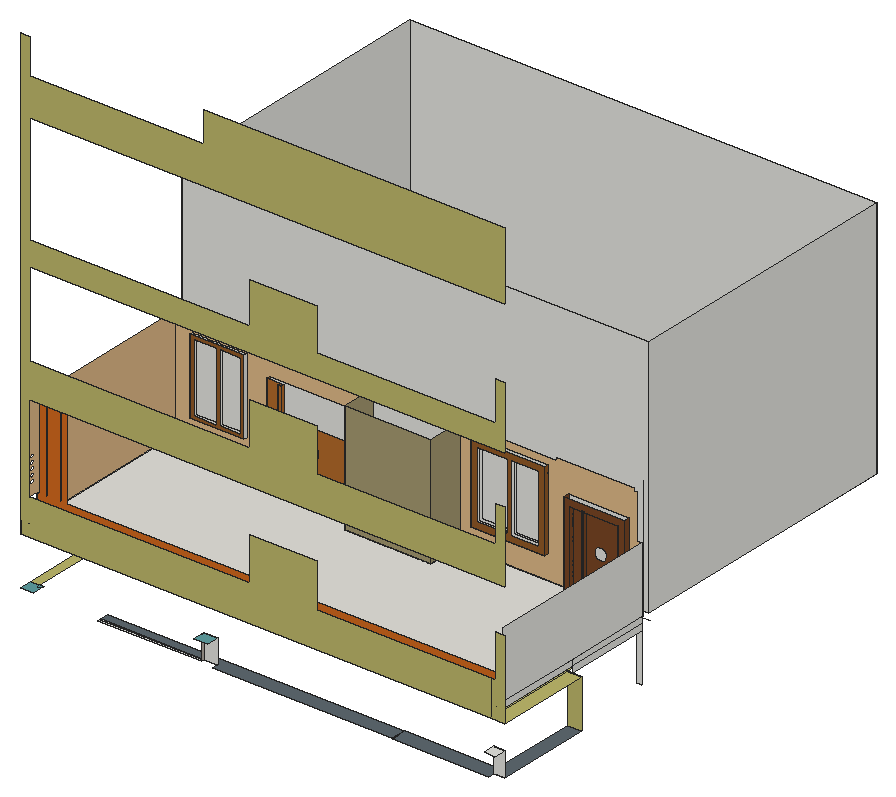
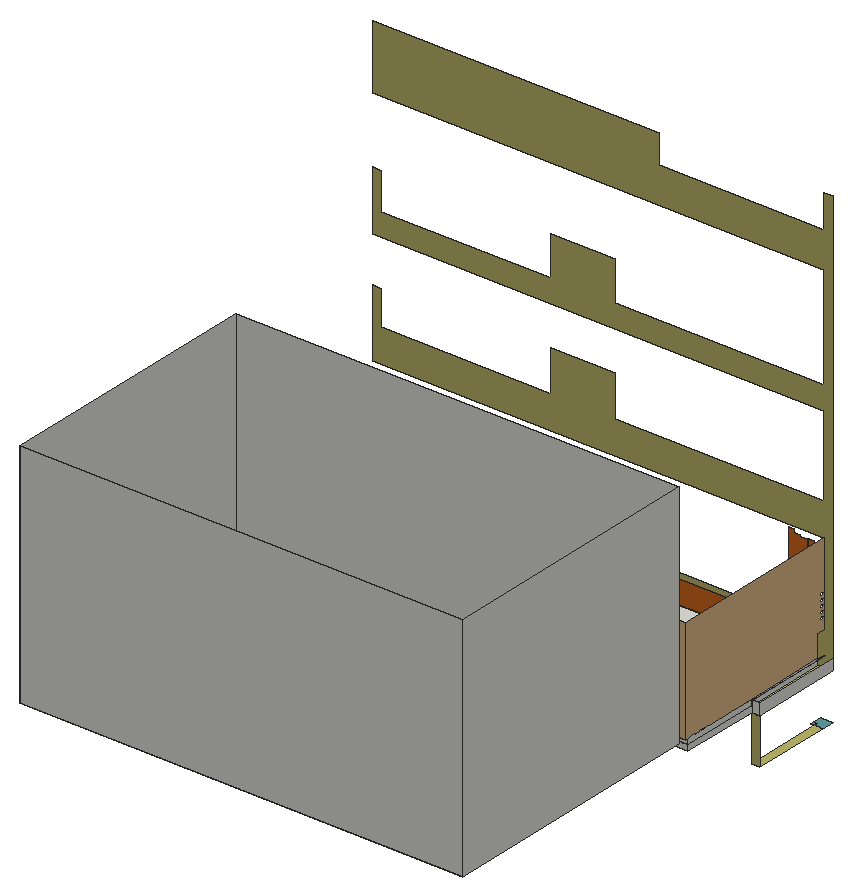
# SketchUp Ruby script. Lengths in inches.
U = 1.inch
M = Sketchup.active_model
def pt(a) = Geom::Point3d.new(a.map { |v| v * U })
def face(e, loops, mat)
  f = e.add_face(loops[0].map { |a| pt(a) })
  loops[1..].each { |l| e.add_face(l.map { |a| pt(a) }).erase! }
  f.material = f.back_material = mat if mat
  f
end
# faces: each face lists its corners as indices into pts; further lists are holes
def faces(e, pts, list, mat = nil) = list.each { |f| face(e, (f[0].is_a?(Array) ? f : [f]).map { |l| l.map { |i| pts[i] } }, mat) }
# xy, xz, yz: faces in a plane at the given z, y or x. An outline is a flat list of corners, or four numbers for a rectangle; further outlines are holes
def ring(l) = l.size == 4 ? [[l[0], l[1]], [l[2], l[1]], [l[2], l[3]], [l[0], l[3]]] : l.each_slice(2).to_a
def flat(e, list, mat, &to3) = list.each { |f| face(e, (f[0].is_a?(Array) ? f : [f]).map { |l| ring(l).map { |u, v| to3.(u, v) } }, mat) }
def xy(e, z, list, mat = nil) = flat(e, list, mat) { |x, y| [x, y, z] }
def xz(e, y, list, mat = nil) = flat(e, list, mat) { |x, z| [x, y, z] }
def yz(e, x, list, mat = nil) = flat(e, list, mat) { |y, z| [x, y, z] }
def lines(e, pts, list) = list.each { |a, b| e.add_line(pt(pts[a]), pt(pts[b])) }
# prism: a flat outline (further loops are holes) pulled along v
def prism(e, loops, v, mat = nil)
  f = face(e, loops, mat); d = Geom::Vector3d.new(v.map { |x| x * U })
  f.pushpull(f.normal.samedirection?(d) ? d.length : -d.length)
end
def box(e, o, s, mat = nil) = prism(e, [[o, [o[0] + s[0], o[1], o[2]], [o[0] + s[0], o[1] + s[1], o[2]], [o[0], o[1] + s[1], o[2]]]], [0, 0, s[2]], mat)
def at(x, y, z, deg = 0) = Geom::Transformation.translation(pt([x, y, z])) * Geom::Transformation.rotation(ORIGIN, Z_AXIS, deg.degrees)
def axes(o, x, y, z) = Geom::Transformation.new([*x, 0, *y, 0, *z, 0, *pt(o).to_a, 1])
def part(name) = M.definitions.add(name)
# library, detail: a bought-in or finely detailed component or shape, given as its bounding box
def library(name, o, s) = part(name).tap { |d| box(d.entities, o, s) }
def detail(e, o, s) = box(e.add_group.entities, o, s)
def put(e, d, t, mat = nil) = e.add_instance(d, t).tap { |i| i.material = mat if mat }
def group(e, t, mat = nil) = e.add_group.tap { |g| g.transformation = t; g.material = mat if mat }.entities
root = M.entities
M.materials.add("[0036_BurlyWood]").color = [222, 184, 135]
M.materials.add("[0041_Chocolate]").color = [210, 105, 30]
M.materials.add("[0057_DarkKhaki]").color = [189, 183, 107]
M.materials.add("[0081_CadetBlue]").color = [95, 158, 160]
M.materials.add("[Formica Speckled Grey]").color = [94, 105, 111]
M.materials.add("[Marble Carrara Gold Floor Tile]").color = [225, 223, 217]
M.materials.add("[Stone Masonry Multi]").color = [182, 175, 164]
M.materials.add("[Translucent Glass Blue]").color = [100, 149, 237]
M.materials["[Translucent Glass Blue]"].alpha = 0.5
M.materials.add("[Wood Bamboo]").color = [177, 105, 43]
M.materials.add("[Wood Floor Parquet]").color = [145, 89, 39]
M.materials.add("[Wood Lumber ButtJoined]").color = [164, 152, 112]
M.materials.add("[Wood Veneer 01]").color = [120, 70, 37]
xy(root,60,[[373.99,6,374.05,12],[79.49,9,181.875,11.375],[79.49,11.375,181.875,12]])
xy(root,60,[[0,24.5,9,106.65]],"[0057_DarkKhaki]")
xy(root,60,[[0,12,12.93,12,12.93,21,9,21,9,24.5,0,24.5],[9,21,12.93,24.5]],"[0081_CadetBlue]")
xy(root,60,[[195.69,6,372.4375,6,372.4375,21,79.49,21,79.49,12,195.69,12],[374.05,6,469.21,6,469.21,12,480,12,480,106.65,466.21,106.65,466.21,21,373.99,21,373.99,12,374.05,12]],"[Formica Speckled Grey]")
xy(root,75.62,[[308.99,189.3,366.74,192.3]])
xy(root,78.62,[[337.87,189.3,341.25,192.3]])
xy(root,78.62,[[311.99,189.3,337.87,192.3],[341.25,189.3,363.74,192.3]],"[Wood Floor Parquet]")
xy(root,84,[[469.21,0,480,12],[246.91,192.3,282.91,196.8]])
xy(root,84,[[181.875,0,195.69,12]],"[0081_CadetBlue]")
xy(root,84,[[246.91,189.3,282.91,192.3]],"[Wood Veneer 01]")
xy(root,88.67,[[242.24,189.3,287.58,192.3]],"[Wood Veneer 01]")
xy(root,89.97,[[341.25,189.3,363.74,192.3]])
xy(root,89.97,[[311.99,189.3,337.87,192.3]],"[Wood Floor Parquet]")
xy(root,92.64,[[311.99,189.3,337.87,192.3],[341.25,189.3,363.74,192.3]],"[Wood Floor Parquet]")
xy(root,101.31,[[337.87,189.3,341.25,192.3],[341.25,189.3,363.74,192.3]])
xy(root,101.31,[[311.99,189.3,337.87,192.3]],"[Wood Floor Parquet]")
xy(root,104.31,[[308.99,189.3,366.74,192.3]])
xy(root,105.6875,[[413.91,189.3,439.47,192.3]],"[Wood Floor Parquet]")
xy(root,108,[[205.37,156.87,290.8125,192.3]])
xy(root,108,[[0,12,0,106.65,9,106.65,9,189.3,90.1,189.3,90.1,186.3,99.83,186.3,99.83,189.3,103.48,189.3,103.48,186.3,113.21,186.3,113.21,189.3,115.97,189.3,115.97,186.3,128.46,186.3,128.46,189.3,186.5,189.3,186.5,192.3,205.37,192.3,205.37,156.87,290.8125,156.87,290.8125,192.3,398.79,192.3,398.79,186.3,405.17,186.3,405.17,189.3,416.3125,189.3,416.3125,186.3,418.65,186.3,418.65,189.3,452.54,189.3,452.54,186.3,458.79,186.3,458.79,192.3,466.21,192.3,466.21,12],[466.21,12,480,106.65]],"[0057_DarkKhaki]")
xy(root,108.6875,[[410.91,189.3,442.47,192.3]])
xy(root,114.1875,[[9,21,471,21,471,192.3,458.79,192.3,458.79,186.3,452.54,186.3,452.54,189.3,418.65,189.3,418.65,186.3,416.3125,186.3,416.3125,189.3,405.17,189.3,405.17,186.3,398.79,186.3,398.79,192.3,290.8125,192.3,290.8125,156.87,205.37,156.87,205.37,192.3,186.5,192.3,186.5,189.3,128.46,189.3,128.46,186.3,115.97,186.3,115.97,189.3,113.21,189.3,113.21,186.3,103.48,186.3,103.48,189.3,99.83,189.3,99.83,186.3,90.1,186.3,90.1,189.3,9,189.3],[205.37,156.87,290.8125,192.3]])
xy(root,120,[[205.37,156.87,290.8125,192.3],[90.1,186.3,99.83,186.3,99.83,189.3,102.5,189.3,102.5,192.3,9,192.3,9,189.3,90.1,189.3],[103.48,186.3,113.21,189.3],[115.97,186.3,118.73,189.3],[118.73,186.3,119.35,189.3],
  [119.35,186.3,128.46,189.3],[398.79,186.3,405.17,192.3],[416.3125,186.3,418.65,186.3,418.65,189.3,452.54,189.3,452.54,192.3,405.17,192.3,405.17,189.3,416.3125,189.3],[452.54,186.3,458.79,192.3],[102.5,189.3,129,192.3],
  [129,189.3,186.5,192.3],[9,201.23,471,483]])
xy(root,120,[[9,21,471,21,471,192.3,458.79,192.3,458.79,186.3,452.54,186.3,452.54,189.3,418.65,189.3,418.65,186.3,416.3125,186.3,416.3125,189.3,405.17,189.3,405.17,186.3,398.79,186.3,398.79,192.3,290.8125,192.3,290.8125,156.87,205.37,156.87,205.37,192.3,186.5,192.3,186.5,189.3,128.46,189.3,128.46,186.3,115.97,186.3,115.97,189.3,113.21,189.3,113.21,186.3,103.48,186.3,103.48,189.3,99.83,189.3,99.83,186.3,90.1,186.3,90.1,189.3,9,189.3]],"[Marble Carrara Gold Floor Tile]")
xy(root,141.78,[[26.52,189.3,79.7,192.3]])
xy(root,143.29,[[303.94,192.3,377.89,195.3]])
xy(root,143.29,[[303.94,189.3,377.89,192.3]],"[Wood Floor Parquet]")
xz(root,12,[[181.875,60,195.69,84],[469.21,60,480,84]])
xz(root,12,[[0,108,466.21,108,466.21,144,293.97,144,293.97,186.625,227.54,186.625,227.54,144,9,144,9,229.6875,480,229.6875,480,300,471,300,471,264,293.97,264,293.97,306.625,227.54,306.625,227.54,264,9,264,9,348,480,348,480,410.4375,471.0625,410.4375,471.0625,372,293.97,372,293.97,413.38,227.54,413.38,227.54,372,9,372,9,480,480,480,480,547.59,181.625,547.59,181.625,517.1875,9,517.1875,9,552,0,552],[466.21,108,480,108,480,186.25,471,186.25,471,144,466.21,144]],"[0057_DarkKhaki]")
xz(root,21,[[9,114.1875,471,120]])
xz(root,21,[[9,120,9,144,12.36,144,12.36,229.6875,17.86,229.6875,17.86,144,20.11,144,20.11,229,25.61,229,25.61,144,26.86,144,26.86,229.6875,32.36,229.6875,32.36,144,33.61,144,33.61,233.5625,39.11,233.5625,39.11,144,471,144,471,120]],"[0041_Chocolate]")
xz(root,106.65,[[0,108,7.75,120],[7.75,108,9,120]])
xz(root,106.65,[[0,60,9,108],[466.21,60,480,108]],"[0057_DarkKhaki]")
xz(root,156.87,[[205.37,108,290.8125,114.1875],[205.37,114.1875,290.8125,120]])
xz(root,156.87,[[205.37,120,290.8125,229.6875]],"[Wood Lumber ButtJoined]")
xz(root,186.3,[[90.1,108,99.83,114.1875],[103.48,108,113.21,114.1875],[115.97,108,118.73,114.1875],[118.73,108,119.35,114.1875],[119.35,108,128.46,114.1875],
  [398.79,108,405.17,114.1875],[416.3125,108,418.65,114.1875],[452.54,108,458.79,114.1875],[90.1,114.1875,99.83,120],[103.48,114.1875,113.21,120],
  [115.97,114.1875,118.73,120],[118.73,114.1875,119.35,120],[119.35,114.1875,128.46,120],[398.79,114.1875,405.17,120],[416.3125,114.1875,418.65,120],
  [452.54,114.1875,458.79,120]])
xz(root,186.3,[[115.97,120,119.35,204],[144.0625,142.74,146.68,143.19,149.1,144.31,151.14,146.01,152.68,148.18,153.6,150.67,153.84,153.32,153.39,155.94,152.28,158.36,150.58,160.4,148.41,161.9375,145.91,162.86,143.26,163.1,140.64,162.65,138.23,161.54,136.18,159.84,134.65,157.67,133.73,155.17,133.48,152.52,133.93,149.9,135.05,147.49,136.75,145.44,138.92,143.91,141.41,142.99]],"[Wood Bamboo]")
xz(root,186.3,[[398.79,120,405.17,120,405.17,197.62,452.41,197.62,452.41,126.38,452.54,120,458.79,120,458.79,204,398.79,204],[416.3125,120,418.65,197.62]],"[Wood Veneer 01]")
xz(root,189.3,[[9,108,90.1,114.1875],[99.83,108,102.5,114.1875],[102.5,108,103.48,114.1875],[113.21,108,115.97,114.1875],[128.46,108,129,114.1875],
  [129,108,186.5,114.1875],[405.17,108,410.91,114.1875],[410.91,108,416.3125,108.6875],[418.65,108,442.47,108.6875],[442.47,108,452.54,114.1875],
  [410.91,108.6875,416.3125,114.1875],[418.65,108.6875,442.47,114.1875],[9,114.1875,90.1,120],[99.83,114.1875,102.5,120],[102.5,114.1875,103.48,120],
  [113.21,114.1875,115.97,120],[128.46,114.1875,129,120],[129,114.1875,186.5,120],[405.17,114.1875,416.3125,120],[418.65,114.1875,452.54,120],
  [115.97,120,119.35,204],[144.0625,142.74,141.41,142.99,138.92,143.91,136.75,145.44,135.05,147.49,133.93,149.9,133.48,152.52,133.73,155.17,134.65,157.67,136.18,159.84,138.23,161.54,140.64,162.65,143.26,163.1,145.91,162.86,148.41,161.9375,150.58,160.4,152.28,158.36,153.39,155.94,153.84,153.32,153.6,150.67,152.68,148.18,151.14,146.01,149.1,144.31,146.68,143.19]])
xz(root,189.3,[[[102.5,120,115.97,204],[112.03,170.25,112.03,173.75,104.03,173.75,104.03,174.75,112.78,174.75,112.78,170.25]],[[119.35,120,186.5,175.57],[144.0625,142.74,141.41,142.99,138.92,143.91,136.75,145.44,135.05,147.49,133.93,149.9,133.48,152.52,133.73,155.17,134.65,157.67,136.18,159.84,138.23,161.54,140.64,162.65,143.26,163.1,145.91,162.86,148.41,161.9375,150.58,160.4,152.28,158.36,153.39,155.94,153.84,153.32,153.6,150.67,152.68,148.18,151.14,146.01,149.1,144.31,146.68,143.19]]],"[Wood Bamboo]")
xz(root,189.3,[[[308.99,75.62,366.74,104.31],[311.99,78.62,363.74,101.31]],[337.87,78.62,341.25,78.62,341.25,89.97,363.74,89.97,363.74,92.64,341.25,92.64,341.25,101.31,337.87,101.31,337.87,92.64,311.99,92.64,311.99,89.97,337.87,89.97],[[26.52,141.78,79.7,216.4],[29.52,144.78,53.11,213.4],[55.4,144.78,76.7,213.4]],[[303.94,143.29,377.89,222.24],[310,149.36,340.91,216.18],[344.375,149.36,371.82,216.18]]],"[Wood Floor Parquet]")
xz(root,189.3,[[405.17,120,416.3125,197.62],[[418.65,120,452.54,120,452.41,126.38,452.41,197.62,418.65,197.62],[433.6,157.54,432,157.57,430.47,158.02,429.1,158.85,428,160.01,427.23,161.41,426.85,162.97,426.89,164.57,427.34,166.1,428.17,167.47,429.32,168.57,430.73,169.34,432.28,169.72,433.88,169.68,435.41,169.23,436.78,168.4,437.88,167.24,438.65,165.84,439.03,164.29,438.99,162.6875,438.54,161.15,437.71,159.79,436.56,158.68,435.15,157.92]]],"[Wood Veneer 01]")
xz(root,192.3,[[466.21,60,471,108],[[308.99,75.62,366.74,104.31],[311.99,78.62,363.74,101.31]],[337.87,78.62,337.87,89.97,311.99,89.97,311.99,92.64,337.87,92.64,337.87,101.31,341.25,101.31,341.25,92.64,363.74,92.64,363.74,89.97,341.25,89.97,341.25,78.62],[186.5,108,205.37,114.1875],[205.37,108,290.8125,114.1875],
  [290.8125,108,398.79,114.1875],[458.79,108,471,114.1875],[186.5,114.1875,205.37,120],[205.37,114.1875,290.8125,120],[290.8125,114.1875,398.79,120],
  [458.79,114.1875,471,120],[102.5,120,186.5,204],[398.79,120,398.79,204,458.79,204,458.79,120,452.54,120,452.41,126.38,452.41,197.62,405.17,197.62,405.17,120],[[26.52,141.78,79.7,216.4],[29.52,144.78,53.11,213.4],[55.4,144.78,76.7,213.4]],[[303.94,143.29,377.89,222.24],[310,149.36,340.91,216.18],[344.375,149.36,371.82,216.18]]])
xz(root,192.3,[[[9,120,102.5,120,102.5,204,186.5,204,186.5,120,205.37,120,205.37,229.6875,184.9,229.6875,184.9,240,100.9,240,100.9,229.6875,9,229.6875],[26.52,141.78,79.7,216.4]],[[290.8125,120,398.79,120,398.79,204,458.79,204,458.79,120,471,120,471,186.25,466.21,186.25,466.21,229.6875,463.09,229.6875,463.09,232.0625,387.22,232.0625,387.22,229.6875,290.8125,229.6875],[303.94,143.29,377.89,222.24]]],"[0036_BurlyWood]")
xz(root,192.3,[[311.99,78.62,337.87,89.97],[341.25,78.62,363.74,89.97],[311.99,92.64,337.87,101.31],[341.25,92.64,363.74,101.31]],"[Translucent Glass Blue]")
xz(root,195.3,[[[303.94,143.29,377.89,222.24],[310,149.36,340.91,216.18],[344.375,149.36,371.82,216.18]]])
xz(root,201.23,[[9,120,471,360]])
xz(root,483,[[9,120,471,360]])
yz(root,0,[[12,108,106.65,120]])
yz(root,9,[[106.65,108,189.3,114.1875],[21,114.1875,106.65,120],[106.65,114.1875,189.3,120],[201.23,120,483,360]])
yz(root,9,[[[21,120,192.3,120,192.3,229.6875,12,229.6875,12,144,21,144],[15.06,176.64,14.51,176.71,13.99,176.92,13.55,177.26,13.21,177.7,13,178.21,12.93,178.76,13,179.3125,13.21,179.82,13.55,180.26,13.99,180.6,14.51,180.8125,15.06,180.89,15.61,180.8125,16.12,180.6,16.56,180.26,16.9,179.82,17.11,179.3125,17.18,178.76,17.11,178.21,16.9,177.7,16.56,177.26,16.12,176.92,15.61,176.71],[15.06,170.95,14.51,171.02,13.99,171.23,13.55,171.57,13.21,172.01,13,172.52,12.93,173.07,13,173.625,13.21,174.14,13.55,174.58,13.99,174.91,14.51,175.125,15.06,175.2,15.61,175.125,16.12,174.91,16.56,174.58,16.9,174.14,17.11,173.625,17.18,173.07,17.11,172.52,16.9,172.01,16.56,171.57,16.12,171.23,15.61,171.02],[15.06,165.26,14.51,165.33,13.99,165.55,13.55,165.88,13.21,166.32,13,166.84,12.93,167.39,13,167.9375,13.21,168.45,13.55,168.89,13.99,169.23,14.51,169.4375,15.06,169.51,15.61,169.4375,16.12,169.23,16.56,168.89,16.9,168.45,17.11,167.9375,17.18,167.39,17.11,166.84,16.9,166.32,16.56,165.88,16.12,165.55,15.61,165.33],[15.06,159.57,14.51,159.65,13.99,159.86,13.55,160.2,13.21,160.64,13,161.15,12.93,161.7,13,162.25,13.21,162.76,13.55,163.2,13.99,163.54,14.51,163.75,15.06,163.82,15.61,163.75,16.12,163.54,16.56,163.2,16.9,162.76,17.11,162.25,17.18,161.7,17.11,161.15,16.9,160.64,16.56,160.2,16.12,159.86,15.61,159.65],[15.06,153.89,14.51,153.96,13.99,154.17,13.55,154.51,13.21,154.95,13,155.46,12.93,156.01,13,156.5625,13.21,157.07,13.55,157.51,13.99,157.85,14.51,158.0625,15.06,158.14,15.61,158.0625,16.12,157.85,16.56,157.51,16.9,157.07,17.11,156.5625,17.18,156.01,17.11,155.46,16.9,154.95,16.56,154.51,16.12,154.17,15.61,153.96]]],"[0036_BurlyWood]")
yz(root,26.52,[[189.3,141.78,192.3,216.4]])
yz(root,79.7,[[189.3,141.78,192.3,216.4]])
yz(root,90.1,[[186.3,108,189.3,114.1875],[186.3,114.1875,189.3,120]])
yz(root,99.83,[[186.3,108,189.3,114.1875],[186.3,114.1875,189.3,120]])
yz(root,102.5,[[189.3,120,192.3,204]],"[Wood Bamboo]")
yz(root,103.48,[[186.3,108,189.3,114.1875],[186.3,114.1875,189.3,120]])
yz(root,113.21,[[186.3,108,189.3,114.1875],[186.3,114.1875,189.3,120]])
yz(root,115.97,[[186.3,108,189.3,114.1875],[186.3,114.1875,189.3,120]])
yz(root,115.97,[[186.3,120,189.3,204]],"[Wood Bamboo]")
yz(root,119.35,[[186.3,120,189.3,204]],"[Wood Bamboo]")
yz(root,128.46,[[186.3,108,189.3,114.1875],[186.3,114.1875,189.3,120]])
yz(root,181.875,[[9,60,12,84]],"[Stone Masonry Multi]")
yz(root,186.5,[[189.3,108,192.3,114.1875],[189.3,114.1875,192.3,120]])
yz(root,186.5,[[189.3,120,192.3,204]],"[Wood Bamboo]")
yz(root,205.37,[[156.87,108,192.3,114.1875],[156.87,114.1875,192.3,120]])
yz(root,205.37,[[156.87,120,192.3,229.6875]],"[Wood Lumber ButtJoined]")
yz(root,290.8125,[[156.87,108,192.3,114.1875],[156.87,114.1875,192.3,120]])
yz(root,290.8125,[[156.87,120,192.3,229.6875]],"[Wood Lumber ButtJoined]")
yz(root,303.94,[[192.3,143.29,195.3,222.24]])
yz(root,303.94,[[189.3,143.29,192.3,222.24]],"[Wood Floor Parquet]")
yz(root,308.99,[[189.3,75.62,192.3,104.31]],"[Wood Floor Parquet]")
yz(root,311.99,[[189.3,89.97,192.3,92.64]])
yz(root,311.99,[[189.3,78.62,192.3,89.97],[189.3,92.64,192.3,101.31]],"[Wood Floor Parquet]")
yz(root,337.87,[[189.3,78.62,192.3,89.97],[189.3,92.64,192.3,101.31]],"[Wood Floor Parquet]")
yz(root,341.25,[[189.3,78.62,192.3,89.97],[189.3,92.64,192.3,101.31]],"[Wood Floor Parquet]")
yz(root,363.74,[[189.3,89.97,192.3,92.64]])
yz(root,363.74,[[189.3,78.62,192.3,89.97],[189.3,92.64,192.3,101.31]],"[Wood Floor Parquet]")
yz(root,366.74,[[189.3,75.62,192.3,104.31]],"[Wood Floor Parquet]")
yz(root,377.89,[[192.3,143.29,195.3,222.24]])
yz(root,377.89,[[189.3,143.29,192.3,222.24]],"[Wood Floor Parquet]")
yz(root,398.79,[[186.3,108,192.3,114.1875],[186.3,114.1875,192.3,120]])
yz(root,398.79,[[186.3,120,192.3,204]],"[Wood Veneer 01]")
yz(root,405.17,[[186.3,108,189.3,114.1875],[186.3,114.1875,189.3,120],[189.3,120,192.3,126.38],[189.3,126.38,192.3,197.62]])
yz(root,405.17,[[186.3,120,189.3,126.38],[186.3,126.38,189.3,197.62]],"[Wood Veneer 01]")
yz(root,416.3125,[[186.3,108,189.3,114.1875],[186.3,114.1875,189.3,120]])
yz(root,416.3125,[[186.3,120,189.3,197.62]],"[Wood Veneer 01]")
yz(root,418.65,[[186.3,108,189.3,114.1875],[186.3,114.1875,189.3,120]])
yz(root,418.65,[[186.3,120,189.3,197.62]],"[Wood Veneer 01]")
yz(root,452.41,[[189.3,126.38,192.3,197.62]])
yz(root,452.41,[[186.3,126.38,189.3,197.62]],"[Wood Veneer 01]")
yz(root,452.54,[[186.3,108,189.3,114.1875],[186.3,114.1875,189.3,120]])
yz(root,458.79,[[186.3,108,192.3,114.1875],[186.3,114.1875,192.3,120]])
yz(root,458.79,[[186.3,120,192.3,204]],"[Wood Veneer 01]")
yz(root,471,[[106.65,108,192.3,114.1875],[21,114.1875,106.65,120],[106.65,114.1875,192.3,120],[21,120,192.3,186.25],[201.23,120,483,360]])
p = [[452.41,186.3,126.38],[452.41,189.3,126.38],[452.54,189.3,120],[452.54,186.3,120],[452.41,192.3,126.38],[452.54,192.3,120],
  [141.41,189.3,142.99],[144.0625,189.3,142.74],[144.0625,186.3,142.74],[141.41,186.3,142.99],[146.68,189.3,143.19],[146.68,186.3,143.19],
  [138.92,189.3,143.91],[138.92,186.3,143.91],[149.1,189.3,144.31],[149.1,186.3,144.31],[471,195.03,120],[471,195.03,240],
  [471,192.3,120],[480,192.3,120],[471,21,114.1875],[471,21,108],[9,21,120],[9,12,120],
  [471,21,120],[471,12,120],[7.75,106.65,120],[7.75,12,120]]
faces(root,p,[[0,1,2,3]],"[Wood Veneer 01]")
faces(root,p,[[4,5,2,1]])
faces(root,p,[[6,7,8,9],[7,10,11,8],[12,6,9,13],[10,14,15,11]],"[Wood Bamboo]")
lines(root,p,[[16,17],[18,19],[16,18],[20,21],[22,23],[24,25],[26,27]])
